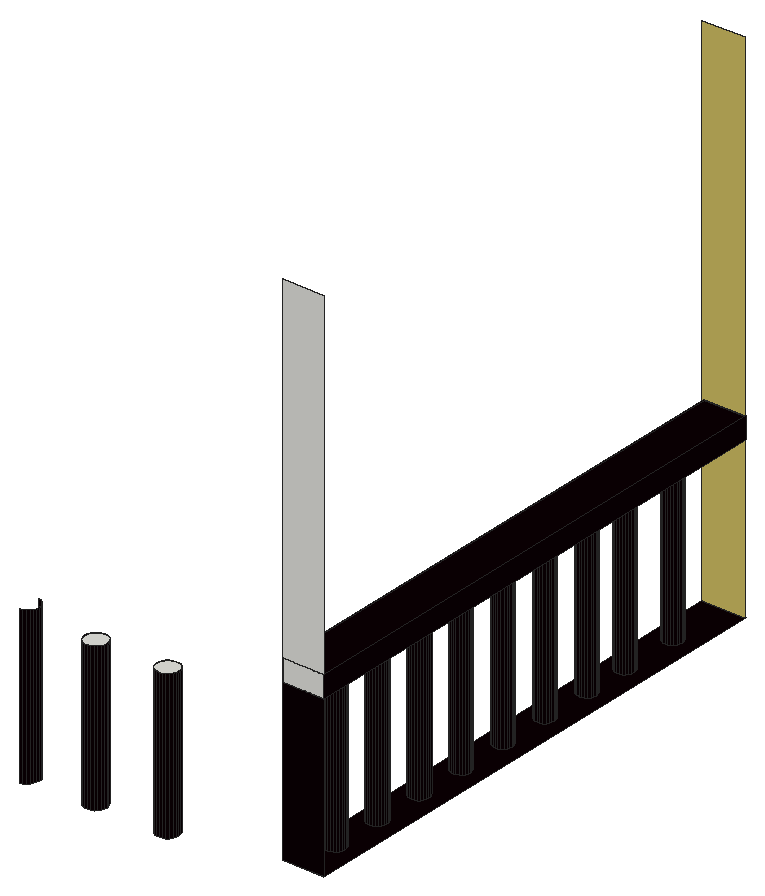
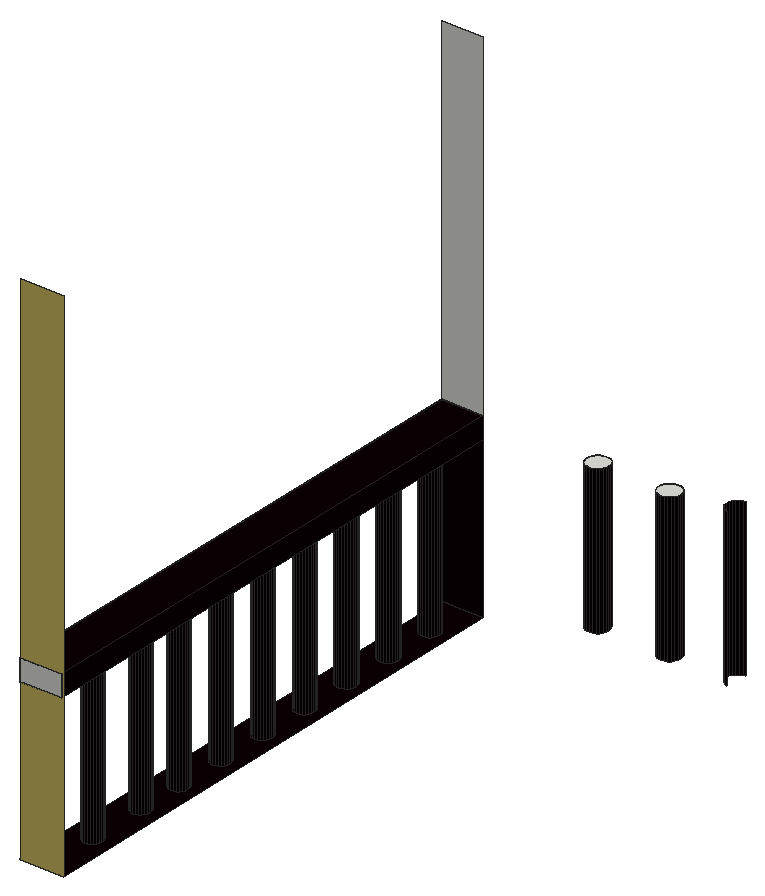
# SketchUp Ruby script. Lengths in inches.
U = 1.inch
M = Sketchup.active_model
def pt(a) = Geom::Point3d.new(a.map { |v| v * U })
def face(e, loops, mat)
  f = e.add_face(loops[0].map { |a| pt(a) })
  loops[1..].each { |l| e.add_face(l.map { |a| pt(a) }).erase! }
  f.material = f.back_material = mat if mat
  f
end
# faces: each face lists its corners as indices into pts; further lists are holes
def faces(e, pts, list, mat = nil) = list.each { |f| face(e, (f[0].is_a?(Array) ? f : [f]).map { |l| l.map { |i| pts[i] } }, mat) }
# xy, xz, yz: faces in a plane at the given z, y or x. An outline is a flat list of corners, or four numbers for a rectangle; further outlines are holes
def ring(l) = l.size == 4 ? [[l[0], l[1]], [l[2], l[1]], [l[2], l[3]], [l[0], l[3]]] : l.each_slice(2).to_a
def flat(e, list, mat, &to3) = list.each { |f| face(e, (f[0].is_a?(Array) ? f : [f]).map { |l| ring(l).map { |u, v| to3.(u, v) } }, mat) }
def xy(e, z, list, mat = nil) = flat(e, list, mat) { |x, y| [x, y, z] }
def xz(e, y, list, mat = nil) = flat(e, list, mat) { |x, z| [x, y, z] }
def yz(e, x, list, mat = nil) = flat(e, list, mat) { |y, z| [x, y, z] }
def lines(e, pts, list) = list.each { |a, b| e.add_line(pt(pts[a]), pt(pts[b])) }
# prism: a flat outline (further loops are holes) pulled along v
def prism(e, loops, v, mat = nil)
  f = face(e, loops, mat); d = Geom::Vector3d.new(v.map { |x| x * U })
  f.pushpull(f.normal.samedirection?(d) ? d.length : -d.length)
end
def box(e, o, s, mat = nil) = prism(e, [[o, [o[0] + s[0], o[1], o[2]], [o[0] + s[0], o[1] + s[1], o[2]], [o[0], o[1] + s[1], o[2]]]], [0, 0, s[2]], mat)
def at(x, y, z, deg = 0) = Geom::Transformation.translation(pt([x, y, z])) * Geom::Transformation.rotation(ORIGIN, Z_AXIS, deg.degrees)
def axes(o, x, y, z) = Geom::Transformation.new([*x, 0, *y, 0, *z, 0, *pt(o).to_a, 1])
def part(name) = M.definitions.add(name)
# library, detail: a bought-in or finely detailed component or shape, given as its bounding box
def library(name, o, s) = part(name).tap { |d| box(d.entities, o, s) }
def detail(e, o, s) = box(e.add_group.entities, o, s)
def put(e, d, t, mat = nil) = e.add_instance(d, t).tap { |i| i.material = mat if mat }
def group(e, t, mat = nil) = e.add_group.tap { |g| g.transformation = t; g.material = mat if mat }.entities
root = M.entities
M.materials.add("[Color D05]").color = [208, 191, 99]
M.materials.add("[Metal Seamed]").color = [11, 0, 4]
xy(root,298.1875,[[559.56,91.34,559.04,91.41,558.56,91.61,558.14,91.92,557.82,92.34,557.625,92.82,557.56,93.34,557.625,93.86,557.82,94.34,558.14,94.75,558.56,95.07,559.04,95.27,559.56,95.34,560.07,95.27,560.56,95.07,560.97,94.75,561.29,94.34,561.49,93.86,561.56,93.34,561.49,92.82,561.29,92.34,560.97,91.92,560.56,91.61,560.07,91.41],[559.56,102.4,559.04,102.47,558.56,102.67,558.14,102.99,557.82,103.4,557.625,103.88,557.56,104.4,557.625,104.92,557.82,105.4,558.14,105.82,558.56,106.13,559.04,106.33,559.56,106.4,560.07,106.33,560.56,106.13,560.97,105.82,561.29,105.4,561.49,104.92,561.56,104.4,561.49,103.88,561.29,103.4,560.97,102.99,560.56,102.67,560.07,102.47],[559.56,113.46,559.04,113.53,558.56,113.73,558.14,114.05,557.82,114.46,557.625,114.95,557.56,115.46,557.625,115.98,557.82,116.46,558.14,116.88,558.56,117.2,559.04,117.4,559.56,117.46,560.07,117.4,560.56,117.2,560.97,116.88,561.29,116.46,561.49,115.98,561.56,115.46,561.49,114.95,561.29,114.46,560.97,114.05,560.56,113.73,560.07,113.53],[559.56,124.53,559.04,124.59,558.56,124.79,558.14,125.11,557.82,125.53,557.625,126.01,557.56,126.53,557.625,127.04,557.82,127.53,558.14,127.94,558.56,128.26,559.04,128.46,559.56,128.53,560.07,128.46,560.56,128.26,560.97,127.94,561.29,127.53,561.49,127.04,561.56,126.53,561.49,126.01,561.29,125.53,560.97,125.11,560.56,124.79,560.07,124.59],[559.56,135.59,559.04,135.66,558.56,135.86,558.14,136.17,557.82,136.59,557.625,137.07,557.56,137.59,557.625,138.11,557.82,138.59,558.14,139,558.56,139.32,559.04,139.52,559.56,139.59,560.07,139.52,560.56,139.32,560.97,139,561.29,138.59,561.49,138.11,561.56,137.59,561.49,137.07,561.29,136.59,560.97,136.17,560.56,135.86,560.07,135.66],
  [559.56,146.65,559.04,146.72,558.56,146.92,558.14,147.24,557.82,147.65,557.625,148.13,557.56,148.65,557.625,149.17,557.82,149.65,558.14,150.07,558.56,150.38,559.04,150.58,559.56,150.65,560.07,150.58,560.56,150.38,560.97,150.07,561.29,149.65,561.49,149.17,561.56,148.65,561.49,148.13,561.29,147.65,560.97,147.24,560.56,146.92,560.07,146.72],[559.56,157.71,559.04,157.78,558.56,157.98,558.14,158.3,557.82,158.71,557.625,159.2,557.56,159.71,557.625,160.23,557.82,160.71,558.14,161.13,558.56,161.45,559.04,161.65,559.56,161.71,560.07,161.65,560.56,161.45,560.97,161.13,561.29,160.71,561.49,160.23,561.56,159.71,561.49,159.2,561.29,158.71,560.97,158.3,560.56,157.98,560.07,157.78],[559.56,167.71,559.04,167.78,558.56,167.98,558.14,168.3,557.82,168.71,557.625,169.2,557.56,169.71,557.625,170.23,557.82,170.71,558.14,171.13,558.56,171.45,559.04,171.65,559.56,171.71,560.07,171.65,560.56,171.45,560.97,171.13,561.29,170.71,561.49,170.23,561.56,169.71,561.49,169.2,561.29,168.71,560.97,168.3,560.56,167.98,560.07,167.78],[559.56,180.4,559.04,180.47,558.56,180.67,558.14,180.99,557.82,181.4,557.625,181.88,557.56,182.4,557.625,182.92,557.82,183.4,558.14,183.82,558.56,184.13,559.04,184.33,559.56,184.4,560.07,184.33,560.56,184.13,560.97,183.82,561.29,183.4,561.49,182.92,561.56,182.4,561.49,181.88,561.29,181.4,560.97,180.99,560.56,180.67,560.07,180.47]])
xy(root,298.1875,[[[555.7,84.18,564.5,84.18,564.5,195.41,555.3125,195.41],[559.56,102.4,559.04,102.47,558.56,102.67,558.14,102.99,557.82,103.4,557.625,103.88,557.56,104.4,557.625,104.92,557.82,105.4,558.14,105.82,558.56,106.13,559.04,106.33,559.56,106.4,560.07,106.33,560.56,106.13,560.97,105.82,561.29,105.4,561.49,104.92,561.56,104.4,561.49,103.88,561.29,103.4,560.97,102.99,560.56,102.67,560.07,102.47],[559.56,113.46,559.04,113.53,558.56,113.73,558.14,114.05,557.82,114.46,557.625,114.95,557.56,115.46,557.625,115.98,557.82,116.46,558.14,116.88,558.56,117.2,559.04,117.4,559.56,117.46,560.07,117.4,560.56,117.2,560.97,116.88,561.29,116.46,561.49,115.98,561.56,115.46,561.49,114.95,561.29,114.46,560.97,114.05,560.56,113.73,560.07,113.53],[559.56,124.53,559.04,124.59,558.56,124.79,558.14,125.11,557.82,125.53,557.625,126.01,557.56,126.53,557.625,127.04,557.82,127.53,558.14,127.94,558.56,128.26,559.04,128.46,559.56,128.53,560.07,128.46,560.56,128.26,560.97,127.94,561.29,127.53,561.49,127.04,561.56,126.53,561.49,126.01,561.29,125.53,560.97,125.11,560.56,124.79,560.07,124.59],[559.56,135.59,559.04,135.66,558.56,135.86,558.14,136.17,557.82,136.59,557.625,137.07,557.56,137.59,557.625,138.11,557.82,138.59,558.14,139,558.56,139.32,559.04,139.52,559.56,139.59,560.07,139.52,560.56,139.32,560.97,139,561.29,138.59,561.49,138.11,561.56,137.59,561.49,137.07,561.29,136.59,560.97,136.17,560.56,135.86,560.07,135.66],[559.56,146.65,559.04,146.72,558.56,146.92,558.14,147.24,557.82,147.65,557.625,148.13,557.56,148.65,557.625,149.17,557.82,149.65,558.14,150.07,558.56,150.38,559.04,150.58,559.56,150.65,560.07,150.58,560.56,150.38,560.97,150.07,561.29,149.65,561.49,149.17,561.56,148.65,561.49,148.13,561.29,147.65,560.97,147.24,560.56,146.92,560.07,146.72],[559.56,157.71,559.04,157.78,558.56,157.98,558.14,158.3,557.82,158.71,557.625,159.2,557.56,159.71,557.625,160.23,557.82,160.71,558.14,161.13,558.56,161.45,559.04,161.65,559.56,161.71,560.07,161.65,560.56,161.45,560.97,161.13,561.29,160.71,561.49,160.23,561.56,159.71,561.49,159.2,561.29,158.71,560.97,158.3,560.56,157.98,560.07,157.78],[559.56,167.71,559.04,167.78,558.56,167.98,558.14,168.3,557.82,168.71,557.625,169.2,557.56,169.71,557.625,170.23,557.82,170.71,558.14,171.13,558.56,171.45,559.04,171.65,559.56,171.71,560.07,171.65,560.56,171.45,560.97,171.13,561.29,170.71,561.49,170.23,561.56,169.71,561.49,169.2,561.29,168.71,560.97,168.3,560.56,167.98,560.07,167.78],[559.56,180.4,559.04,180.47,558.56,180.67,558.14,180.99,557.82,181.4,557.625,181.88,557.56,182.4,557.625,182.92,557.82,183.4,558.14,183.82,558.56,184.13,559.04,184.33,559.56,184.4,560.07,184.33,560.56,184.13,560.97,183.82,561.29,183.4,561.49,182.92,561.56,182.4,561.49,181.88,561.29,181.4,560.97,180.99,560.56,180.67,560.07,180.47],[559.56,91.34,559.04,91.41,558.56,91.61,558.14,91.92,557.82,92.34,557.625,92.82,557.56,93.34,557.625,93.86,557.82,94.34,558.14,94.75,558.56,95.07,559.04,95.27,559.56,95.34,560.07,95.27,560.56,95.07,560.97,94.75,561.29,94.34,561.49,93.86,561.56,93.34,561.49,92.82,561.29,92.34,560.97,91.92,560.56,91.61,560.07,91.41]]],"[Metal Seamed]")
xy(root,300,[[521.97,74.99,521.36,75.05,520.8,75.25,520.3,75.6,519.91,76.06,519.66,76.61,519.55,77.2,519.6,77.8,519.81,78.37,520.16,78.86,520.62,79.25,521.16,79.51,521.76,79.61,522.36,79.5625,522.93,79.36,523.42,79.01,523.8125,78.55,524.07,78,524.17,77.41,524.12,76.81,523.91,76.24,523.57,75.74,523.11,75.36,522.56,75.1],[537.09,74.99,536.49,75.05,535.92,75.25,535.43,75.6,535.04,76.06,534.78,76.61,534.68,77.2,534.73,77.8,534.94,78.37,535.28,78.86,535.74,79.25,536.29,79.51,536.88,79.61,537.49,79.5625,538.05,79.36,538.55,79.01,538.9375,78.55,539.19,78,539.3,77.41,539.25,76.81,539.04,76.24,538.69,75.74,538.23,75.36,537.69,75.1]])
xy(root,331.0625,[[521.97,74.99,522.56,75.1,523.11,75.36,523.57,75.74,523.91,76.24,524.12,76.81,524.17,77.41,524.07,78,523.8125,78.55,523.42,79.01,522.93,79.36,522.36,79.5625,521.76,79.61,521.16,79.51,520.62,79.25,520.16,78.86,519.81,78.37,519.6,77.8,519.55,77.2,519.66,76.61,519.91,76.06,520.3,75.6,520.8,75.25,521.36,75.05]])
xy(root,331.125,[[537.09,74.99,537.69,75.1,538.23,75.36,538.69,75.74,539.04,76.24,539.25,76.81,539.3,77.41,539.19,78,538.9375,78.55,538.55,79.01,538.05,79.36,537.49,79.5625,536.88,79.61,536.29,79.51,535.74,79.25,535.28,78.86,534.94,78.37,534.73,77.8,534.68,77.2,534.78,76.61,535.04,76.06,535.43,75.6,535.92,75.25,536.49,75.05]])
xy(root,331.82,[[[555.7,84.18,564.5,195.41],[559.56,124.53,560.07,124.59,560.56,124.79,560.97,125.11,561.29,125.53,561.49,126.01,561.56,126.53,561.49,127.04,561.29,127.53,560.97,127.94,560.56,128.26,560.07,128.46,559.56,128.53,559.04,128.46,558.56,128.26,558.14,127.94,557.82,127.53,557.625,127.04,557.56,126.53,557.625,126.01,557.82,125.53,558.14,125.11,558.56,124.79,559.04,124.59],[559.56,180.4,560.07,180.47,560.56,180.67,560.97,180.99,561.29,181.4,561.49,181.88,561.56,182.4,561.49,182.92,561.29,183.4,560.97,183.82,560.56,184.13,560.07,184.33,559.56,184.4,559.04,184.33,558.56,184.13,558.14,183.82,557.82,183.4,557.625,182.92,557.56,182.4,557.625,181.88,557.82,181.4,558.14,180.99,558.56,180.67,559.04,180.47]]])
xy(root,332.125,[[559.56,113.46,560.07,113.53,560.56,113.73,560.97,114.05,561.29,114.46,561.49,114.95,561.56,115.46,561.49,115.98,561.29,116.46,560.97,116.88,560.56,117.2,560.07,117.4,559.56,117.46,559.04,117.4,558.56,117.2,558.14,116.88,557.82,116.46,557.625,115.98,557.56,115.46,557.625,114.95,557.82,114.46,558.14,114.05,558.56,113.73,559.04,113.53]])
xy(root,332.1875,[[559.56,91.34,560.07,91.41,560.56,91.61,560.97,91.92,561.29,92.34,561.49,92.82,561.56,93.34,561.49,93.86,561.29,94.34,560.97,94.75,560.56,95.07,560.07,95.27,559.56,95.34,559.04,95.27,558.56,95.07,558.14,94.75,557.82,94.34,557.625,93.86,557.56,93.34,557.625,92.82,557.82,92.34,558.14,91.92,558.56,91.61,559.04,91.41]])
xy(root,332.3125,[[559.56,157.71,560.07,157.78,560.56,157.98,560.97,158.3,561.29,158.71,561.49,159.2,561.56,159.71,561.49,160.23,561.29,160.71,560.97,161.13,560.56,161.45,560.07,161.65,559.56,161.71,559.04,161.65,558.56,161.45,558.14,161.13,557.82,160.71,557.625,160.23,557.56,159.71,557.625,159.2,557.82,158.71,558.14,158.3,558.56,157.98,559.04,157.78]])
xy(root,332.4375,[[559.56,167.71,560.07,167.78,560.56,167.98,560.97,168.3,561.29,168.71,561.49,169.2,561.56,169.71,561.49,170.23,561.29,170.71,560.97,171.13,560.56,171.45,560.07,171.65,559.56,171.71,559.04,171.65,558.56,171.45,558.14,171.13,557.82,170.71,557.625,170.23,557.56,169.71,557.625,169.2,557.82,168.71,558.14,168.3,558.56,167.98,559.04,167.78]])
xy(root,332.75,[[559.56,102.4,560.07,102.47,560.56,102.67,560.97,102.99,561.29,103.4,561.49,103.88,561.56,104.4,561.49,104.92,561.29,105.4,560.97,105.82,560.56,106.13,560.07,106.33,559.56,106.4,559.04,106.33,558.56,106.13,558.14,105.82,557.82,105.4,557.625,104.92,557.56,104.4,557.625,103.88,557.82,103.4,558.14,102.99,558.56,102.67,559.04,102.47]])
xy(root,333.1875,[[559.56,135.59,560.07,135.66,560.56,135.86,560.97,136.17,561.29,136.59,561.49,137.07,561.56,137.59,561.49,138.11,561.29,138.59,560.97,139,560.56,139.32,560.07,139.52,559.56,139.59,559.04,139.52,558.56,139.32,558.14,139,557.82,138.59,557.625,138.11,557.56,137.59,557.625,137.07,557.82,136.59,558.14,136.17,558.56,135.86,559.04,135.66]])
xy(root,333.625,[[559.56,146.65,560.07,146.72,560.56,146.92,560.97,147.24,561.29,147.65,561.49,148.13,561.56,148.65,561.49,149.17,561.29,149.65,560.97,150.07,560.56,150.38,560.07,150.58,559.56,150.65,559.04,150.58,558.56,150.38,558.14,150.07,557.82,149.65,557.625,149.17,557.56,148.65,557.625,148.13,557.82,147.65,558.14,147.24,558.56,146.92,559.04,146.72]])
xy(root,336.35,[[555.7,84.18,564.5,195.41]],"[Metal Seamed]")
xz(root,84.18,[[555.7,331.82,564.5,336.35],[555.7,336.35,564.5,408]])
xz(root,84.18,[[555.7,298.1875,564.5,331.82]],"[Metal Seamed]")
xz(root,195.41,[[555.7,331.82,564.3125,336.35],[564.3125,331.82,564.5,336.35]])
xz(root,195.41,[[555.3125,298.1875,564.3125,298.1875,564.3125,331.82,555.7,331.82,555.7,336.35,564.3125,336.35,564.3125,408,555.3125,408]],"[Color D05]")
yz(root,555.7,[[84.18,331.82,195.41,336.35]],"[Metal Seamed]")
yz(root,564.5,[[84.18,331.82,195.41,336.35]],"[Metal Seamed]")
p = [[559.04,91.41,298.1875],[559.56,91.34,298.1875],[559.56,91.34,332.1875],[559.04,91.41,332.1875],[560.07,91.41,298.1875],[560.07,91.41,332.1875],
  [558.56,91.61,298.1875],[558.56,91.61,332.1875],[560.56,91.61,298.1875],[560.56,91.61,332.1875],[558.14,91.92,298.1875],[558.14,91.92,332.1875],
  [560.97,91.92,298.1875],[560.97,91.92,332.1875],[557.82,92.34,298.1875],[557.82,92.34,332.1875],[561.29,92.34,298.1875],[561.29,92.34,332.1875],
  [557.625,92.82,298.1875],[557.625,92.82,332.1875],[561.49,92.82,298.1875],[561.49,92.82,332.1875],[557.56,93.34,298.1875],[557.56,93.34,332.1875],
  [561.56,93.34,298.1875],[561.56,93.34,332.1875],[557.625,93.86,298.1875],[557.625,93.86,332.1875],[561.49,93.86,298.1875],[561.49,93.86,332.1875],
  [557.82,94.34,298.1875],[557.82,94.34,332.1875],[561.29,94.34,298.1875],[561.29,94.34,332.1875],[558.14,94.75,298.1875],[558.14,94.75,332.1875],
  [560.97,94.75,298.1875],[560.97,94.75,332.1875],[558.56,95.07,298.1875],[558.56,95.07,332.1875],[560.56,95.07,298.1875],[560.56,95.07,332.1875],
  [559.04,95.27,298.1875],[559.04,95.27,332.1875],[560.07,95.27,298.1875],[560.07,95.27,332.1875],[559.56,95.34,298.1875],[559.56,95.34,332.1875],
  [559.04,102.47,298.1875],[559.56,102.4,298.1875],[559.56,102.4,332.75],[559.04,102.47,332.75],[560.07,102.47,298.1875],[560.07,102.47,332.75],
  [558.56,102.67,298.1875],[558.56,102.67,332.75],[560.56,102.67,298.1875],[560.56,102.67,332.75],[558.14,102.99,298.1875],[558.14,102.99,332.75],
  [560.97,102.99,298.1875],[560.97,102.99,332.75],[557.82,103.4,298.1875],[557.82,103.4,332.75],[561.29,103.4,298.1875],[561.29,103.4,332.75],
  [557.625,103.88,298.1875],[557.625,103.88,332.75],[561.49,103.88,298.1875],[561.49,103.88,332.75],[557.56,104.4,298.1875],[557.56,104.4,332.75],
  [561.56,104.4,298.1875],[561.56,104.4,332.75],[557.625,104.92,298.1875],[557.625,104.92,332.75],[561.49,104.92,298.1875],[561.49,104.92,332.75],
  [557.82,105.4,298.1875],[557.82,105.4,332.75],[561.29,105.4,298.1875],[561.29,105.4,332.75],[558.14,105.82,298.1875],[558.14,105.82,332.75],
  [560.97,105.82,298.1875],[560.97,105.82,332.75],[558.56,106.13,298.1875],[558.56,106.13,332.75],[560.56,106.13,298.1875],[560.56,106.13,332.75],
  [559.04,106.33,298.1875],[559.04,106.33,332.75],[560.07,106.33,298.1875],[560.07,106.33,332.75],[559.56,106.4,298.1875],[559.56,106.4,332.75],
  [558.56,113.73,298.1875],[559.04,113.53,298.1875],[559.04,113.53,332.125],[558.56,113.73,332.125],[559.56,113.46,298.1875],[559.56,113.46,332.125],
  [560.07,113.53,298.1875],[560.07,113.53,332.125],[560.56,113.73,298.1875],[560.56,113.73,332.125],[558.14,114.05,298.1875],[558.14,114.05,332.125],
  [560.97,114.05,298.1875],[560.97,114.05,332.125],[557.82,114.46,298.1875],[557.82,114.46,332.125],[561.29,114.46,298.1875],[561.29,114.46,332.125],
  [557.625,114.95,298.1875],[557.625,114.95,332.125],[561.49,114.95,298.1875],[561.49,114.95,332.125],[557.56,115.46,298.1875],[557.56,115.46,332.125],
  [561.56,115.46,298.1875],[561.56,115.46,332.125],[557.625,115.98,298.1875],[557.625,115.98,332.125],[561.49,115.98,298.1875],[561.49,115.98,332.125],
  [557.82,116.46,298.1875],[557.82,116.46,332.125],[561.29,116.46,298.1875],[561.29,116.46,332.125],[558.14,116.88,298.1875],[558.14,116.88,332.125],
  [560.97,116.88,298.1875],[560.97,116.88,332.125],[558.56,117.2,298.1875],[558.56,117.2,332.125],[560.56,117.2,298.1875],[560.56,117.2,332.125],
  [559.04,117.4,298.1875],[559.04,117.4,332.125],[560.07,117.4,298.1875],[560.07,117.4,332.125],[559.56,117.46,298.1875],[559.56,117.46,332.125],
  [559.04,124.59,298.1875],[559.56,124.53,298.1875],[559.56,124.53,331.82],[559.04,124.59,331.82],[560.07,124.59,298.1875],[560.07,124.59,331.82],
  [558.56,124.79,298.1875],[558.56,124.79,331.82],[560.56,124.79,298.1875],[560.56,124.79,331.82],[558.14,125.11,298.1875],[558.14,125.11,331.82],
  [560.97,125.11,298.1875],[560.97,125.11,331.82],[557.82,125.53,298.1875],[557.82,125.53,331.82],[561.29,125.53,298.1875],[561.29,125.53,331.82],
  [557.625,126.01,298.1875],[557.625,126.01,331.82],[561.49,126.01,298.1875],[561.49,126.01,331.82],[557.56,126.53,298.1875],[557.56,126.53,331.82],
  [561.56,126.53,298.1875],[561.56,126.53,331.82],[557.625,127.04,298.1875],[557.625,127.04,331.82],[561.49,127.04,298.1875],[561.49,127.04,331.82],
  [557.82,127.53,298.1875],[557.82,127.53,331.82],[561.29,127.53,298.1875],[561.29,127.53,331.82],[558.14,127.94,298.1875],[558.14,127.94,331.82],
  [560.97,127.94,298.1875],[560.97,127.94,331.82],[558.56,128.26,298.1875],[558.56,128.26,331.82],[560.56,128.26,298.1875],[560.56,128.26,331.82],
  [559.04,128.46,298.1875],[559.04,128.46,331.82],[560.07,128.46,298.1875],[560.07,128.46,331.82],[559.56,128.53,298.1875],[559.56,128.53,331.82],
  [559.04,135.66,298.1875],[559.56,135.59,298.1875],[559.56,135.59,333.1875],[559.04,135.66,333.1875],[560.07,135.66,298.1875],[560.07,135.66,333.1875],
  [558.56,135.86,298.1875],[558.56,135.86,333.1875],[560.56,135.86,298.1875],[560.56,135.86,333.1875],[558.14,136.17,298.1875],[558.14,136.17,333.1875],
  [560.97,136.17,298.1875],[560.97,136.17,333.1875],[557.82,136.59,298.1875],[557.82,136.59,333.1875],[561.29,136.59,298.1875],[561.29,136.59,333.1875],
  [557.625,137.07,298.1875],[557.625,137.07,333.1875],[561.49,137.07,298.1875],[561.49,137.07,333.1875],[557.56,137.59,298.1875],[557.56,137.59,333.1875],
  [561.56,137.59,298.1875],[561.56,137.59,333.1875],[557.625,138.11,298.1875],[557.625,138.11,333.1875],[561.49,138.11,298.1875],[561.49,138.11,333.1875],
  [557.82,138.59,298.1875],[557.82,138.59,333.1875],[561.29,138.59,298.1875],[561.29,138.59,333.1875],[558.14,139,298.1875],[558.14,139,333.1875],
  [560.97,139,298.1875],[560.97,139,333.1875],[558.56,139.32,298.1875],[558.56,139.32,333.1875],[560.56,139.32,298.1875],[560.56,139.32,333.1875],
  [559.04,139.52,298.1875],[559.04,139.52,333.1875],[560.07,139.52,298.1875],[560.07,139.52,333.1875],[559.56,139.59,298.1875],[559.56,139.59,333.1875],
  [558.56,146.92,298.1875],[559.04,146.72,298.1875],[559.04,146.72,333.625],[558.56,146.92,333.625],[559.56,146.65,298.1875],[559.56,146.65,333.625],
  [560.07,146.72,298.1875],[560.07,146.72,333.625],[560.56,146.92,298.1875],[560.56,146.92,333.625],[558.14,147.24,298.1875],[558.14,147.24,333.625],
  [560.97,147.24,298.1875],[560.97,147.24,333.625],[557.82,147.65,298.1875],[557.82,147.65,333.625],[561.29,147.65,298.1875],[561.29,147.65,333.625],
  [557.625,148.13,298.1875],[557.625,148.13,333.625],[561.49,148.13,298.1875],[561.49,148.13,333.625],[557.56,148.65,298.1875],[557.56,148.65,333.625],
  [561.56,148.65,298.1875],[561.56,148.65,333.625],[557.625,149.17,298.1875],[557.625,149.17,333.625],[561.49,149.17,298.1875],[561.49,149.17,333.625],
  [557.82,149.65,298.1875],[557.82,149.65,333.625],[561.29,149.65,298.1875],[561.29,149.65,333.625],[558.14,150.07,298.1875],[558.14,150.07,333.625],
  [560.97,150.07,298.1875],[560.97,150.07,333.625],[558.56,150.38,298.1875],[558.56,150.38,333.625],[560.56,150.38,298.1875],[560.56,150.38,333.625],
  [559.04,150.58,298.1875],[559.04,150.58,333.625],[560.07,150.58,298.1875],[560.07,150.58,333.625],[559.56,150.65,298.1875],[559.56,150.65,333.625],
  [559.04,157.78,298.1875],[559.56,157.71,298.1875],[559.56,157.71,332.3125],[559.04,157.78,332.3125],[560.07,157.78,298.1875],[560.07,157.78,332.3125],
  [558.56,157.98,298.1875],[558.56,157.98,332.3125],[560.56,157.98,298.1875],[560.56,157.98,332.3125],[558.14,158.3,298.1875],[558.14,158.3,332.3125],
  [560.97,158.3,298.1875],[560.97,158.3,332.3125],[557.82,158.71,298.1875],[557.82,158.71,332.3125],[561.29,158.71,298.1875],[561.29,158.71,332.3125],
  [557.625,159.2,298.1875],[557.625,159.2,332.3125],[561.49,159.2,298.1875],[561.49,159.2,332.3125],[557.56,159.71,298.1875],[557.56,159.71,332.3125],
  [561.56,159.71,298.1875],[561.56,159.71,332.3125],[557.625,160.23,298.1875],[557.625,160.23,332.3125],[561.49,160.23,298.1875],[561.49,160.23,332.3125],
  [557.82,160.71,298.1875],[557.82,160.71,332.3125],[561.29,160.71,298.1875],[561.29,160.71,332.3125],[558.14,161.13,298.1875],[558.14,161.13,332.3125],
  [560.97,161.13,298.1875],[560.97,161.13,332.3125],[558.56,161.45,298.1875],[558.56,161.45,332.3125],[560.56,161.45,298.1875],[560.56,161.45,332.3125],
  [559.04,161.65,298.1875],[559.04,161.65,332.3125],[560.07,161.65,298.1875],[560.07,161.65,332.3125],[559.56,161.71,298.1875],[559.56,161.71,332.3125],
  [559.04,167.78,298.1875],[559.56,167.71,298.1875],[559.56,167.71,332.4375],[559.04,167.78,332.4375],[560.07,167.78,298.1875],[560.07,167.78,332.4375],
  [558.56,167.98,298.1875],[558.56,167.98,332.4375],[560.56,167.98,298.1875],[560.56,167.98,332.4375],[558.14,168.3,298.1875],[558.14,168.3,332.4375],
  [560.97,168.3,298.1875],[560.97,168.3,332.4375],[557.82,168.71,298.1875],[557.82,168.71,332.4375],[561.29,168.71,298.1875],[561.29,168.71,332.4375],
  [557.625,169.2,298.1875],[557.625,169.2,332.4375],[561.49,169.2,298.1875],[561.49,169.2,332.4375],[557.56,169.71,298.1875],[557.56,169.71,332.4375],
  [561.56,169.71,298.1875],[561.56,169.71,332.4375],[557.625,170.23,298.1875],[557.625,170.23,332.4375],[561.49,170.23,298.1875],[561.49,170.23,332.4375],
  [557.82,170.71,298.1875],[557.82,170.71,332.4375],[561.29,170.71,298.1875],[561.29,170.71,332.4375],[558.14,171.13,298.1875],[558.14,171.13,332.4375],
  [560.97,171.13,298.1875],[560.97,171.13,332.4375],[558.56,171.45,298.1875],[558.56,171.45,332.4375],[560.56,171.45,298.1875],[560.56,171.45,332.4375],
  [559.04,171.65,298.1875],[559.04,171.65,332.4375],[560.07,171.65,298.1875],[560.07,171.65,332.4375],[559.56,171.71,298.1875],[559.56,171.71,332.4375],
  [559.04,180.47,298.1875],[559.56,180.4,298.1875],[559.56,180.4,331.82],[559.04,180.47,331.82],[560.07,180.47,298.1875],[560.07,180.47,331.82],
  [558.56,180.67,298.1875],[558.56,180.67,331.82],[560.56,180.67,298.1875],[560.56,180.67,331.82],[558.14,180.99,298.1875],[558.14,180.99,331.82],
  [560.97,180.99,298.1875],[560.97,180.99,331.82],[557.82,181.4,298.1875],[557.82,181.4,331.82],[561.29,181.4,298.1875],[561.29,181.4,331.82],
  [557.625,181.88,298.1875],[557.625,181.88,331.82],[561.49,181.88,298.1875],[561.49,181.88,331.82],[557.56,182.4,298.1875],[557.56,182.4,331.82],
  [561.56,182.4,298.1875],[561.56,182.4,331.82],[557.625,182.92,298.1875],[557.625,182.92,331.82],[561.49,182.92,298.1875],[561.49,182.92,331.82],
  [557.82,183.4,298.1875],[557.82,183.4,331.82],[561.29,183.4,298.1875],[561.29,183.4,331.82],[558.14,183.82,298.1875],[558.14,183.82,331.82],
  [560.97,183.82,298.1875],[560.97,183.82,331.82],[558.56,184.13,298.1875],[558.56,184.13,331.82],[560.56,184.13,298.1875],[560.56,184.13,331.82],
  [559.04,184.33,298.1875],[559.04,184.33,331.82],[560.07,184.33,298.1875],[560.07,184.33,331.82],[559.56,184.4,298.1875],[559.56,184.4,331.82],
  [507.65,74.99,300],[508.25,75.1,300],[508.25,75.1,332.875],[507.65,74.99,332.875],[520.8,75.25,300],[521.36,75.05,300],
  [521.36,75.05,331.0625],[520.8,75.25,331.0625],[521.97,74.99,300],[521.97,74.99,331.0625],[522.56,75.1,300],[522.56,75.1,331.0625],
  [535.92,75.25,300],[536.49,75.05,300],[536.49,75.05,331.125],[535.92,75.25,331.125],[537.09,74.99,300],[537.09,74.99,331.125],
  [537.69,75.1,300],[537.69,75.1,331.125],[508.79,75.36,300],[508.79,75.36,332.875],[523.11,75.36,300],[523.11,75.36,331.0625],
  [538.23,75.36,300],[538.23,75.36,331.125],[520.3,75.6,300],[520.3,75.6,331.0625],[535.43,75.6,300],[535.43,75.6,331.125],
  [509.26,75.74,300],[509.26,75.74,332.875],[523.57,75.74,300],[523.57,75.74,331.0625],[538.69,75.74,300],[538.69,75.74,331.125],
  [519.91,76.06,300],[519.91,76.06,331.0625],[535.04,76.06,300],[535.04,76.06,331.125],[509.6,76.24,300],[509.6,76.24,332.875],
  [523.91,76.24,300],[523.91,76.24,331.0625],[539.04,76.24,300],[539.04,76.24,331.125],[519.66,76.61,300],[519.66,76.61,331.0625],
  [534.78,76.61,300],[534.78,76.61,331.125],[509.81,76.81,300],[509.81,76.81,332.875],[524.12,76.81,300],[524.12,76.81,331.0625],
  [539.25,76.81,300],[539.25,76.81,331.125],[519.55,77.2,300],[519.55,77.2,331.0625],[534.68,77.2,300],[534.68,77.2,331.125],
  [509.86,77.41,300],[509.86,77.41,332.875],[524.17,77.41,300],[524.17,77.41,331.0625],[539.3,77.41,300],[539.3,77.41,331.125],
  [519.6,77.8,300],[519.6,77.8,331.0625],[534.73,77.8,300],[534.73,77.8,331.125],[509.75,78,300],[509.75,78,332.875],
  [524.07,78,300],[524.07,78,331.0625],[539.19,78,300],[539.19,78,331.125],[519.81,78.37,300],[519.81,78.37,331.0625],
  [534.94,78.37,300],[534.94,78.37,331.125],[509.5,78.55,300],[509.5,78.55,332.875],[523.8125,78.55,300],[523.8125,78.55,331.0625],
  [538.9375,78.55,300],[538.9375,78.55,331.125],[520.16,78.86,300],[520.16,78.86,331.0625],[535.28,78.86,300],[535.28,78.86,331.125],
  [509.11,79.01,300],[509.11,79.01,332.875],[523.42,79.01,300],[523.42,79.01,331.0625],[538.55,79.01,300],[538.55,79.01,331.125],
  [520.62,79.25,300],[520.62,79.25,331.0625],[535.74,79.25,300],[535.74,79.25,331.125],[508.62,79.36,300],[508.62,79.36,332.875],
  [522.93,79.36,300],[522.93,79.36,331.0625],[538.05,79.36,300],[538.05,79.36,331.125],[521.16,79.51,300],[521.16,79.51,331.0625],
  [536.29,79.51,300],[536.29,79.51,331.125],[508.05,79.5625,300],[508.05,79.5625,332.875],[522.36,79.5625,300],[522.36,79.5625,331.0625],
  [537.49,79.5625,300],[537.49,79.5625,331.125],[521.76,79.61,300],[521.76,79.61,331.0625],[536.88,79.61,300],[536.88,79.61,331.125]]
faces(root,p,[[0,1,2,3],[1,4,5,2],[6,0,3,7],[4,8,9,5],[10,6,7,11],[8,12,13,9],[14,10,11,15],[12,16,17,13],
  [18,14,15,19],[16,20,21,17],[22,18,19,23],[20,24,25,21],[26,22,23,27],[24,28,29,25],[30,26,27,31],[28,32,33,29],
  [34,30,31,35],[32,36,37,33],[38,34,35,39],[36,40,41,37],[42,38,39,43],[40,44,45,41],[46,42,43,47],[44,46,47,45],
  [48,49,50,51],[49,52,53,50],[54,48,51,55],[52,56,57,53],[58,54,55,59],[56,60,61,57],[62,58,59,63],[60,64,65,61],
  [66,62,63,67],[64,68,69,65],[70,66,67,71],[68,72,73,69],[74,70,71,75],[72,76,77,73],[78,74,75,79],[76,80,81,77],
  [82,78,79,83],[80,84,85,81],[86,82,83,87],[84,88,89,85],[90,86,87,91],[88,92,93,89],[94,90,91,95],[92,94,95,93],
  [96,97,98,99],[97,100,101,98],[100,102,103,101],[102,104,105,103],[106,96,99,107],[104,108,109,105],[110,106,107,111],[108,112,113,109],
  [114,110,111,115],[112,116,117,113],[118,114,115,119],[116,120,121,117],[122,118,119,123],[120,124,125,121],[126,122,123,127],[124,128,129,125],
  [130,126,127,131],[128,132,133,129],[134,130,131,135],[132,136,137,133],[138,134,135,139],[136,140,141,137],[142,138,139,143],[140,142,143,141],
  [144,145,146,147],[145,148,149,146],[150,144,147,151],[148,152,153,149],[154,150,151,155],[152,156,157,153],[158,154,155,159],[156,160,161,157],
  [162,158,159,163],[160,164,165,161],[166,162,163,167],[164,168,169,165],[170,166,167,171],[168,172,173,169],[174,170,171,175],[172,176,177,173],
  [178,174,175,179],[176,180,181,177],[182,178,179,183],[180,184,185,181],[186,182,183,187],[184,188,189,185],[190,186,187,191],[188,190,191,189],
  [192,193,194,195],[193,196,197,194],[198,192,195,199],[196,200,201,197],[202,198,199,203],[200,204,205,201],[206,202,203,207],[204,208,209,205],
  [210,206,207,211],[208,212,213,209],[214,210,211,215],[212,216,217,213],[218,214,215,219],[216,220,221,217],[222,218,219,223],[220,224,225,221],
  [226,222,223,227],[224,228,229,225],[230,226,227,231],[228,232,233,229],[234,230,231,235],[232,236,237,233],[238,234,235,239],[236,238,239,237],
  [240,241,242,243],[241,244,245,242],[244,246,247,245],[246,248,249,247],[250,240,243,251],[248,252,253,249],[254,250,251,255],[252,256,257,253],
  [258,254,255,259],[256,260,261,257],[262,258,259,263],[260,264,265,261],[266,262,263,267],[264,268,269,265],[270,266,267,271],[268,272,273,269],
  [274,270,271,275],[272,276,277,273],[278,274,275,279],[276,280,281,277],[282,278,279,283],[280,284,285,281],[286,282,283,287],[284,286,287,285],
  [288,289,290,291],[289,292,293,290],[294,288,291,295],[292,296,297,293],[298,294,295,299],[296,300,301,297],[302,298,299,303],[300,304,305,301],
  [306,302,303,307],[304,308,309,305],[310,306,307,311],[308,312,313,309],[314,310,311,315],[312,316,317,313],[318,314,315,319],[316,320,321,317],
  [322,318,319,323],[320,324,325,321],[326,322,323,327],[324,328,329,325],[330,326,327,331],[328,332,333,329],[334,330,331,335],[332,334,335,333],
  [336,337,338,339],[337,340,341,338],[342,336,339,343],[340,344,345,341],[346,342,343,347],[344,348,349,345],[350,346,347,351],[348,352,353,349],
  [354,350,351,355],[352,356,357,353],[358,354,355,359],[356,360,361,357],[362,358,359,363],[360,364,365,361],[366,362,363,367],[364,368,369,365],
  [370,366,367,371],[368,372,373,369],[374,370,371,375],[372,376,377,373],[378,374,375,379],[376,380,381,377],[382,378,379,383],[380,382,383,381],
  [384,385,386,387],[385,388,389,386],[390,384,387,391],[388,392,393,389],[394,390,391,395],[392,396,397,393],[398,394,395,399],[396,400,401,397],
  [402,398,399,403],[400,404,405,401],[406,402,403,407],[404,408,409,405],[410,406,407,411],[408,412,413,409],[414,410,411,415],[412,416,417,413],
  [418,414,415,419],[416,420,421,417],[422,418,419,423],[420,424,425,421],[426,422,423,427],[424,428,429,425],[430,426,427,431],[428,430,431,429],
  [432,433,434,435],[436,437,438,439],[437,440,441,438],[440,442,443,441],[444,445,446,447],[445,448,449,446],[448,450,451,449],[433,452,453,434],
  [442,454,455,443],[450,456,457,451],[458,436,439,459],[460,444,447,461],[452,462,463,453],[454,464,465,455],[456,466,467,457],[468,458,459,469],
  [470,460,461,471],[462,472,473,463],[464,474,475,465],[466,476,477,467],[478,468,469,479],[480,470,471,481],[472,482,483,473],[474,484,485,475],
  [476,486,487,477],[488,478,479,489],[490,480,481,491],[482,492,493,483],[484,494,495,485],[486,496,497,487],[498,488,489,499],[500,490,491,501],
  [492,502,503,493],[494,504,505,495],[496,506,507,497],[508,498,499,509],[510,500,501,511],[502,512,513,503],[504,514,515,505],[506,516,517,507],
  [518,508,509,519],[520,510,511,521],[512,522,523,513],[514,524,525,515],[516,526,527,517],[528,518,519,529],[530,520,521,531],[522,532,533,523],
  [524,534,535,525],[526,536,537,527],[538,528,529,539],[540,530,531,541],[532,542,543,533],[534,544,545,535],[536,546,547,537],[548,538,539,549],
  [550,540,541,551],[544,548,549,545],[546,550,551,547]],"[Metal Seamed]")
